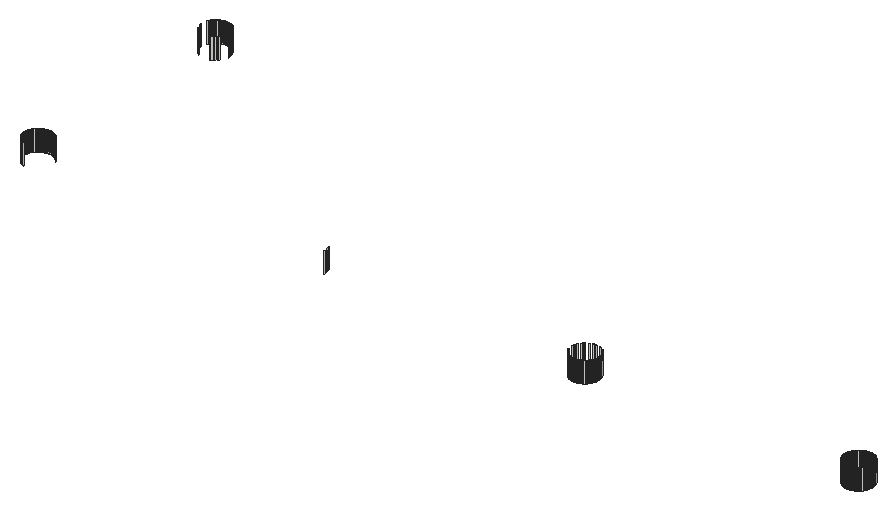
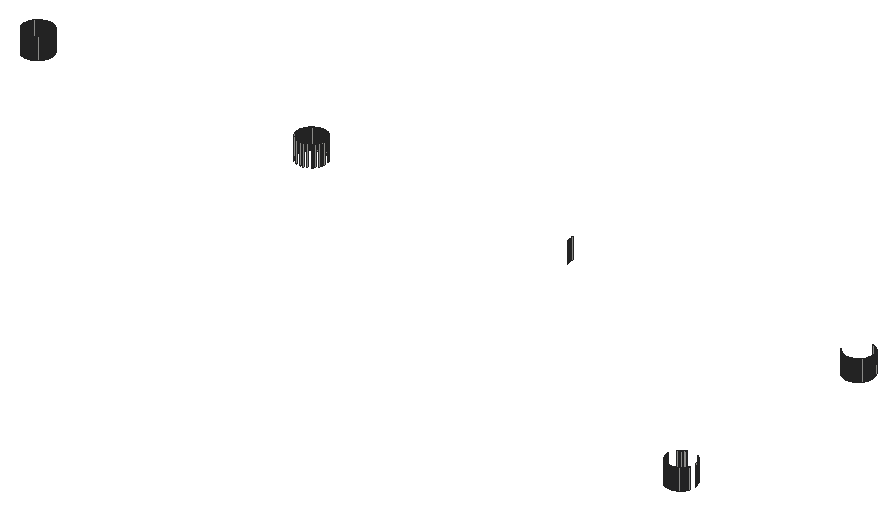
# SketchUp Ruby script. Lengths in millimetres.
U = 1.mm
M = Sketchup.active_model
def pt(a) = Geom::Point3d.new(a.map { |v| v * U })
def face(e, loops, mat)
  f = e.add_face(loops[0].map { |a| pt(a) })
  loops[1..].each { |l| e.add_face(l.map { |a| pt(a) }).erase! }
  f.material = f.back_material = mat if mat
  f
end
# faces: each face lists its corners as indices into pts; further lists are holes
def faces(e, pts, list, mat = nil) = list.each { |f| face(e, (f[0].is_a?(Array) ? f : [f]).map { |l| l.map { |i| pts[i] } }, mat) }
# xy, xz, yz: faces in a plane at the given z, y or x. An outline is a flat list of corners, or four numbers for a rectangle; further outlines are holes
def ring(l) = l.size == 4 ? [[l[0], l[1]], [l[2], l[1]], [l[2], l[3]], [l[0], l[3]]] : l.each_slice(2).to_a
def flat(e, list, mat, &to3) = list.each { |f| face(e, (f[0].is_a?(Array) ? f : [f]).map { |l| ring(l).map { |u, v| to3.(u, v) } }, mat) }
def xy(e, z, list, mat = nil) = flat(e, list, mat) { |x, y| [x, y, z] }
def xz(e, y, list, mat = nil) = flat(e, list, mat) { |x, z| [x, y, z] }
def yz(e, x, list, mat = nil) = flat(e, list, mat) { |y, z| [x, y, z] }
def lines(e, pts, list) = list.each { |a, b| e.add_line(pt(pts[a]), pt(pts[b])) }
# prism: a flat outline (further loops are holes) pulled along v
def prism(e, loops, v, mat = nil)
  f = face(e, loops, mat); d = Geom::Vector3d.new(v.map { |x| x * U })
  f.pushpull(f.normal.samedirection?(d) ? d.length : -d.length)
end
def box(e, o, s, mat = nil) = prism(e, [[o, [o[0] + s[0], o[1], o[2]], [o[0] + s[0], o[1] + s[1], o[2]], [o[0], o[1] + s[1], o[2]]]], [0, 0, s[2]], mat)
def at(x, y, z, deg = 0) = Geom::Transformation.translation(pt([x, y, z])) * Geom::Transformation.rotation(ORIGIN, Z_AXIS, deg.degrees)
def axes(o, x, y, z) = Geom::Transformation.new([*x, 0, *y, 0, *z, 0, *pt(o).to_a, 1])
def part(name) = M.definitions.add(name)
# library, detail: a bought-in or finely detailed component or shape, given as its bounding box
def library(name, o, s) = part(name).tap { |d| box(d.entities, o, s) }
def detail(e, o, s) = box(e.add_group.entities, o, s)
def put(e, d, t, mat = nil) = e.add_instance(d, t).tap { |i| i.material = mat if mat }
def group(e, t, mat = nil) = e.add_group.tap { |g| g.transformation = t; g.material = mat if mat }.entities
root = M.entities
p = [[2470.7,177.9,2718.2],[2470.7,177.9,2794],[2473.9,177.8,2794],[2473.9,177.8,2718.2],[2477.1,177.9,2794],[2477.1,177.9,2718.2],
  [3479,177.9,2718.2],[3479,177.9,2794],[3482.2,177.8,2794],[3482.2,177.8,2718.2],[3485.4,177.9,2794],[3485.4,177.9,2718.2],
  [2467.5,178.2,2718.2],[2467.5,178.2,2794],[2480.2,178.2,2794],[2480.2,178.2,2718.2],[3475.8,178.2,2718.2],[3475.8,178.2,2794],
  [3488.6,178.2,2794],[3488.6,178.2,2718.2],[2464.3,178.7,2718.2],[2464.3,178.7,2794],[2483.4,178.7,2794],[2483.4,178.7,2718.2],
  [3472.7,178.7,2718.2],[3472.7,178.7,2794],[3491.7,178.7,2794],[3491.7,178.7,2718.2],[2461.2,179.4,2718.2],[2461.2,179.4,2794],
  [2486.5,179.4,2794],[2486.5,179.4,2718.2],[3469.6,179.4,2718.2],[3469.6,179.4,2794],[3494.8,179.4,2794],[3494.8,179.4,2718.2],
  [444.6,179.4,2794],[444.6,179.4,2718.2],[441.5,180.3,2718.2],[441.5,180.3,2794],[2458.2,180.3,2718.2],[2458.2,180.3,2794],
  [2489.6,180.3,2794],[2489.6,180.3,2718.2],[3466.5,180.3,2718.2],[3466.5,180.3,2794],[3497.9,180.3,2794],[3497.9,180.3,2718.2],
  [438.5,181.4,2718.2],[438.5,181.4,2794],[2455.2,181.4,2718.2],[2455.2,181.4,2794],[2492.6,181.4,2794],[2492.6,181.4,2718.2],
  [3463.5,181.4,2718.2],[3463.5,181.4,2794],[3500.9,181.4,2794],[3500.9,181.4,2718.2],[435.6,182.6,2718.2],[435.6,182.6,2794],
  [2452.2,182.6,2718.2],[2452.2,182.6,2794],[2495.5,182.6,2794],[2495.5,182.6,2718.2],[3460.6,182.6,2718.2],[3460.6,182.6,2794],
  [3503.8,182.6,2794],[3503.8,182.6,2718.2],[432.7,184.1,2718.2],[432.7,184.1,2794],[2449.4,184.1,2718.2],[2449.4,184.1,2794],
  [2498.3,184.1,2794],[2498.3,184.1,2718.2],[3457.7,184.1,2718.2],[3457.7,184.1,2794],[3506.7,184.1,2794],[3506.7,184.1,2718.2],
  [430,185.7,2718.2],[430,185.7,2794],[2446.6,185.7,2718.2],[2446.6,185.7,2794],[2501.1,185.7,2794],[2501.1,185.7,2718.2],
  [3455,185.7,2718.2],[3455,185.7,2794],[3509.4,185.7,2794],[3509.4,185.7,2718.2],[427.3,187.5,2718.2],[427.3,187.5,2794],
  [2444,187.5,2718.2],[2444,187.5,2794],[2503.7,187.5,2794],[2503.7,187.5,2718.2],[3452.3,187.5,2718.2],[3452.3,187.5,2794],
  [3512.1,187.5,2794],[3512.1,187.5,2718.2],[424.8,189.5,2718.2],[424.8,189.5,2794],[2441.5,189.5,2718.2],[2441.5,189.5,2794],
  [2506.2,189.5,2794],[2506.2,189.5,2718.2],[3449.8,189.5,2718.2],[3449.8,189.5,2794],[3514.6,189.5,2794],[3514.6,189.5,2718.2],
  [422.4,191.6,2718.2],[422.4,191.6,2794],[2439.1,191.6,2718.2],[2439.1,191.6,2794],[2508.6,191.6,2794],[2508.6,191.6,2718.2],
  [3447.4,191.6,2718.2],[3447.4,191.6,2794],[3517,191.6,2794],[3517,191.6,2718.2],[420.2,193.8,2718.2],[420.2,193.8,2794],
  [2436.8,193.8,2718.2],[2436.8,193.8,2794],[2510.9,193.8,2794],[2510.9,193.8,2718.2],[3445.2,193.8,2718.2],[3445.2,193.8,2794],
  [3519.2,193.8,2794],[3519.2,193.8,2718.2],[418.1,196.2,2718.2],[418.1,196.2,2794],[2434.7,196.2,2718.2],[2434.7,196.2,2794],
  [2513,196.2,2794],[2513,196.2,2718.2],[3443.1,196.2,2718.2],[3443.1,196.2,2794],[3521.3,196.2,2794],[3521.3,196.2,2718.2],
  [416.1,198.7,2718.2],[416.1,198.7,2794],[2432.8,198.7,2718.2],[2432.8,198.7,2794],[2515,198.7,2794],[2515,198.7,2718.2],
  [3441.1,198.7,2718.2],[3441.1,198.7,2794],[3523.3,198.7,2794],[3523.3,198.7,2718.2],[414.3,201.4,2718.2],[414.3,201.4,2794],
  [2431,201.4,2718.2],[2431,201.4,2794],[2516.8,201.4,2794],[2516.8,201.4,2718.2],[3439.3,201.4,2718.2],[3439.3,201.4,2794],
  [3525.1,201.4,2794],[3525.1,201.4,2718.2],[412.7,204.1,2718.2],[412.7,204.1,2794],[2429.4,204.1,2718.2],[2429.4,204.1,2794],
  [2518.4,204.1,2794],[2518.4,204.1,2718.2],[3437.7,204.1,2718.2],[3437.7,204.1,2794],[3526.7,204.1,2794],[3526.7,204.1,2718.2],
  [411.2,207,2718.2],[411.2,207,2794],[2427.9,207,2718.2],[2427.9,207,2794],[2519.8,207,2794],[2519.8,207,2718.2],
  [3436.2,207,2718.2],[3436.2,207,2794],[3528.2,207,2794],[3528.2,207,2718.2],[410,209.9,2718.2],[410,209.9,2794],
  [2426.6,209.9,2718.2],[2426.6,209.9,2794],[2521.1,209.9,2794],[2521.1,209.9,2718.2],[3435,209.9,2718.2],[3435,209.9,2794],
  [3529.4,209.9,2794],[3529.4,209.9,2718.2],[408.9,212.9,2718.2],[408.9,212.9,2794],[2425.6,212.9,2718.2],[2425.6,212.9,2794],
  [2522.2,212.9,2794],[2522.2,212.9,2718.2],[3433.9,212.9,2718.2],[3433.9,212.9,2794],[3530.5,212.9,2794],[3530.5,212.9,2718.2],
  [408,216,2718.2],[408,216,2794],[2523.1,216,2794],[2523.1,216,2718.2],[3433,216,2718.2],[3433,216,2794],
  [3531.4,216,2794],[3531.4,216,2718.2],[407.3,219.1,2718.2],[407.3,219.1,2794],[2523.8,219.1,2794],[2523.8,219.1,2718.2],
  [3432.3,219.1,2718.2],[3432.3,219.1,2794],[3532.1,219.1,2794],[3532.1,219.1,2718.2],[406.8,222.2,2718.2],[406.8,222.2,2794],
  [2524.3,222.2,2794],[2524.3,222.2,2718.2],[3431.8,222.2,2718.2],[3431.8,222.2,2794],[3532.6,222.2,2794],[3532.6,222.2,2718.2],
  [406.5,225.4,2718.2],[406.5,225.4,2794],[1516.2,225.4,2794],[1516.2,225.4,2718.2],[1515.9,222.2,2718.2],[1515.9,222.2,2794],
  [2524.6,225.4,2794],[2524.6,225.4,2718.2],[3431.5,225.4,2718.2],[3431.5,225.4,2794],[3532.9,225.4,2794],[3532.9,225.4,2718.2],
  [406.4,228.6,2718.2],[406.4,228.6,2794],[2524.7,228.6,2794],[2524.7,228.6,2718.2],[3431.4,228.6,2718.2],[3431.4,228.6,2794],
  [3533,228.6,2794],[3533,228.6,2718.2],[406.5,231.8,2718.2],[406.5,231.8,2794],[2524.6,231.8,2794],[2524.6,231.8,2718.2],
  [3431.5,231.8,2718.2],[3431.5,231.8,2794],[3532.9,231.8,2794],[3532.9,231.8,2718.2],[406.8,235,2718.2],[406.8,235,2794],
  [2423.2,231.8,2794],[2423.2,231.8,2718.2],[2423.5,235,2718.2],[2423.5,235,2794],[2524.3,235,2794],[2524.3,235,2718.2],
  [3431.8,235,2718.2],[3431.8,235,2794],[3532.6,235,2794],[3532.6,235,2718.2],[407.3,238.1,2718.2],[407.3,238.1,2794],
  [2424,238.1,2718.2],[2424,238.1,2794],[2523.8,238.1,2794],[2523.8,238.1,2718.2],[3432.3,238.1,2718.2],[3432.3,238.1,2794],
  [3532.1,238.1,2794],[3532.1,238.1,2718.2],[408,241.2,2718.2],[408,241.2,2794],[1514.7,241.2,2794],[1514.7,241.2,2718.2],
  [1515.4,238.1,2718.2],[1515.4,238.1,2794],[2424.7,241.2,2718.2],[2424.7,241.2,2794],[2523.1,241.2,2794],[2523.1,241.2,2718.2],
  [3433,241.2,2718.2],[3433,241.2,2794],[3531.4,241.2,2794],[3531.4,241.2,2718.2],[408.9,244.3,2718.2],[408.9,244.3,2794],
  [1513.8,244.3,2794],[1513.8,244.3,2718.2],[2522.2,244.3,2794],[2522.2,244.3,2718.2],[3433.9,244.3,2718.2],[3433.9,244.3,2794],
  [3530.5,244.3,2794],[3530.5,244.3,2718.2],[410,247.3,2718.2],[410,247.3,2794],[1512.8,247.3,2794],[1512.8,247.3,2718.2],
  [2521.1,247.3,2794],[2521.1,247.3,2718.2],[3435,247.3,2718.2],[3435,247.3,2794],[3529.4,247.3,2794],[3529.4,247.3,2718.2],
  [411.2,250.2,2718.2],[411.2,250.2,2794],[1511.5,250.2,2794],[1511.5,250.2,2718.2],[2426.6,247.3,2794],[2426.6,247.3,2718.2],
  [2427.9,250.2,2718.2],[2427.9,250.2,2794],[2519.8,250.2,2794],[2519.8,250.2,2718.2],[3436.2,250.2,2718.2],[3436.2,250.2,2794],
  [3528.2,250.2,2794],[3528.2,250.2,2718.2],[412.7,253.1,2718.2],[412.7,253.1,2794],[2518.4,253.1,2794],[2518.4,253.1,2718.2],
  [3437.7,253.1,2718.2],[3437.7,253.1,2794],[3526.7,253.1,2794],[3526.7,253.1,2718.2],[414.3,255.8,2718.2],[414.3,255.8,2794],
  [500.1,255.8,2794],[500.1,255.8,2718.2],[501.7,253.1,2718.2],[501.7,253.1,2794],[3439.3,255.8,2718.2],[3439.3,255.8,2794],
  [3525.1,255.8,2794],[3525.1,255.8,2718.2],[416.1,258.5,2718.2],[416.1,258.5,2794],[498.3,258.5,2794],[498.3,258.5,2718.2],
  [3441.1,258.5,2718.2],[3441.1,258.5,2794],[3523.3,258.5,2794],[3523.3,258.5,2718.2],[418.1,261,2718.2],[418.1,261,2794],
  [496.3,261,2794],[496.3,261,2718.2],[2432.8,258.5,2794],[2432.8,258.5,2718.2],[2434.7,261,2718.2],[2434.7,261,2794],
  [3443.1,261,2718.2],[3443.1,261,2794],[3521.3,261,2794],[3521.3,261,2718.2],[420.2,263.4,2718.2],[420.2,263.4,2794],
  [494.2,263.4,2794],[494.2,263.4,2718.2],[2436.8,263.4,2718.2],[2436.8,263.4,2794],[3445.2,263.4,2718.2],[3445.2,263.4,2794],
  [3519.2,263.4,2794],[3519.2,263.4,2718.2],[422.4,265.6,2718.2],[422.4,265.6,2794],[492,265.6,2794],[492,265.6,2718.2],
  [2439.1,265.6,2718.2],[2439.1,265.6,2794],[3447.4,265.6,2718.2],[3447.4,265.6,2794],[3517,265.6,2794],[3517,265.6,2718.2],
  [424.8,267.7,2718.2],[424.8,267.7,2794],[489.6,267.7,2794],[489.6,267.7,2718.2],[2441.5,267.7,2718.2],[2441.5,267.7,2794],
  [2506.2,267.7,2794],[2506.2,267.7,2718.2],[2508.6,265.6,2718.2],[2508.6,265.6,2794],[3449.8,267.7,2718.2],[3449.8,267.7,2794],
  [3514.6,267.7,2794],[3514.6,267.7,2718.2],[427.3,269.7,2718.2],[427.3,269.7,2794],[487.1,269.7,2794],[487.1,269.7,2718.2],
  [3452.3,269.7,2718.2],[3452.3,269.7,2794],[3512.1,269.7,2794],[3512.1,269.7,2718.2],[430,271.5,2718.2],[430,271.5,2794],
  [484.4,271.5,2794],[484.4,271.5,2718.2],[3455,271.5,2718.2],[3455,271.5,2794],[3509.4,271.5,2794],[3509.4,271.5,2718.2],
  [432.7,273.1,2718.2],[432.7,273.1,2794],[481.7,273.1,2794],[481.7,273.1,2718.2],[3457.7,273.1,2718.2],[3457.7,273.1,2794],
  [3506.7,273.1,2794],[3506.7,273.1,2718.2],[435.6,274.6,2718.2],[435.6,274.6,2794],[478.8,274.6,2794],[478.8,274.6,2718.2],
  [3460.6,274.6,2718.2],[3460.6,274.6,2794],[3503.8,274.6,2794],[3503.8,274.6,2718.2],[438.5,275.8,2718.2],[438.5,275.8,2794],
  [475.9,275.8,2794],[475.9,275.8,2718.2],[2452.2,274.6,2794],[2452.2,274.6,2718.2],[2455.2,275.8,2718.2],[2455.2,275.8,2794],
  [3463.5,275.8,2718.2],[3463.5,275.8,2794],[3500.9,275.8,2794],[3500.9,275.8,2718.2],[441.5,276.9,2718.2],[441.5,276.9,2794],
  [472.9,276.9,2794],[472.9,276.9,2718.2],[2489.6,276.9,2794],[2489.6,276.9,2718.2],[2492.6,275.8,2718.2],[2492.6,275.8,2794],
  [3466.5,276.9,2718.2],[3466.5,276.9,2794],[3497.9,276.9,2794],[3497.9,276.9,2718.2],[444.6,277.8,2718.2],[444.6,277.8,2794],
  [469.8,277.8,2794],[469.8,277.8,2718.2],[3469.6,277.8,2718.2],[3469.6,277.8,2794],[3494.8,277.8,2794],[3494.8,277.8,2718.2],
  [447.7,278.5,2718.2],[447.7,278.5,2794],[466.7,278.5,2794],[466.7,278.5,2718.2],[2461.2,277.8,2794],[2461.2,277.8,2718.2],
  [2464.3,278.5,2718.2],[2464.3,278.5,2794],[3472.7,278.5,2718.2],[3472.7,278.5,2794],[3491.7,278.5,2794],[3491.7,278.5,2718.2],
  [450.8,279,2718.2],[450.8,279,2794],[463.6,279,2794],[463.6,279,2718.2],[2467.5,279,2718.2],[2467.5,279,2794],
  [3475.8,279,2718.2],[3475.8,279,2794],[3488.6,279,2794],[3488.6,279,2718.2],[454,279.3,2718.2],[454,279.3,2794],
  [460.4,279.3,2794],[460.4,279.3,2718.2],[3479,279.3,2718.2],[3479,279.3,2794],[3485.4,279.3,2794],[3485.4,279.3,2718.2],
  [457.2,279.4,2718.2],[457.2,279.4,2794],[2473.9,279.4,2794],[2473.9,279.4,2718.2],[2477.1,279.3,2718.2],[2477.1,279.3,2794],
  [3482.2,279.4,2718.2],[3482.2,279.4,2794],[475.9,999,2718.2],[475.9,999,2794],[478.8,1000.3,2794],[478.8,1000.3,2718.2],
  [481.7,1001.8,2794],[481.7,1001.8,2718.2],[430,1003.4,2718.2],[430,1003.4,2794],[432.7,1001.8,2794],[432.7,1001.8,2718.2],
  [427.3,1005.2,2718.2],[427.3,1005.2,2794],[484.4,1003.4,2718.2],[484.4,1003.4,2794],[487.1,1005.2,2794],[487.1,1005.2,2718.2],
  [489.6,1007.1,2794],[489.6,1007.1,2718.2],[422.4,1009.2,2718.2],[422.4,1009.2,2794],[424.8,1007.1,2794],[424.8,1007.1,2718.2],
  [420.2,1011.5,2718.2],[420.2,1011.5,2794],[494.2,1011.5,2718.2],[494.2,1011.5,2794],[496.3,1013.9,2794],[496.3,1013.9,2718.2],
  [416.1,1016.4,2718.2],[416.1,1016.4,2794],[418.1,1013.9,2794],[418.1,1013.9,2718.2],[498.3,1016.4,2794],[498.3,1016.4,2718.2],
  [414.3,1019,2718.2],[414.3,1019,2794],[407.3,1036.7,2718.2],[407.3,1036.7,2794],[408,1033.6,2794],[408,1033.6,2718.2],
  [406.8,1039.9,2718.2],[406.8,1039.9,2794],[507.9,1043.1,2718.2],[507.9,1043.1,2794],[508,1046.3,2794],[508,1046.3,2718.2],
  [507.9,1049.5,2794],[507.9,1049.5,2718.2],[507.6,1052.6,2794],[507.6,1052.6,2718.2],[507.1,1055.8,2794],[507.1,1055.8,2718.2],
  [506.4,1058.9,2794],[506.4,1058.9,2718.2],[505.5,1062,2794],[505.5,1062,2718.2],[504.4,1065,2794],[504.4,1065,2718.2],
  [411.2,1067.9,2718.2],[411.2,1067.9,2794],[410,1065,2794],[410,1065,2718.2],[412.7,1070.7,2718.2],[412.7,1070.7,2794],
  [414.3,1073.5,2718.2],[414.3,1073.5,2794],[501.7,1070.7,2718.2],[501.7,1070.7,2794],[500.1,1073.5,2794],[500.1,1073.5,2718.2],
  [416.1,1076.1,2718.2],[416.1,1076.1,2794],[498.3,1076.1,2794],[498.3,1076.1,2718.2],[418.1,1078.6,2718.2],[418.1,1078.6,2794],
  [496.3,1078.6,2794],[496.3,1078.6,2718.2],[420.2,1081,2718.2],[420.2,1081,2794],[494.2,1081,2794],[494.2,1081,2718.2],
  [422.4,1083.3,2718.2],[422.4,1083.3,2794],[492,1083.3,2794],[492,1083.3,2718.2],[424.8,1085.4,2718.2],[424.8,1085.4,2794],
  [489.6,1085.4,2794],[489.6,1085.4,2718.2],[427.3,1087.4,2718.2],[427.3,1087.4,2794],[487.1,1087.4,2794],[487.1,1087.4,2718.2],
  [430,1089.2,2718.2],[430,1089.2,2794],[484.4,1089.2,2794],[484.4,1089.2,2718.2],[432.7,1090.8,2718.2],[432.7,1090.8,2794],
  [481.7,1090.8,2794],[481.7,1090.8,2718.2],[435.6,1092.2,2718.2],[435.6,1092.2,2794],[478.8,1092.2,2794],[478.8,1092.2,2718.2],
  [438.5,1093.5,2718.2],[438.5,1093.5,2794],[475.9,1093.5,2794],[475.9,1093.5,2718.2],[441.5,1094.6,2718.2],[441.5,1094.6,2794],
  [472.9,1094.6,2794],[472.9,1094.6,2718.2],[444.6,1095.5,2718.2],[444.6,1095.5,2794],[469.8,1095.5,2794],[469.8,1095.5,2718.2],
  [447.7,1096.2,2718.2],[447.7,1096.2,2794],[466.7,1096.2,2794],[466.7,1096.2,2718.2],[450.8,1096.7,2718.2],[450.8,1096.7,2794],
  [463.6,1096.7,2794],[463.6,1096.7,2718.2],[454,1097,2718.2],[454,1097,2794],[460.4,1097,2794],[460.4,1097,2718.2],
  [457.2,1097.1,2718.2],[457.2,1097.1,2794]]
faces(root,p,[[0,1,2,3],[3,2,4,5],[6,7,8,9],[9,8,10,11],[12,13,1,0],[5,4,14,15],[16,17,7,6],[11,10,18,19],
  [20,21,13,12],[15,14,22,23],[24,25,17,16],[19,18,26,27],[28,29,21,20],[23,22,30,31],[32,33,25,24],[27,26,34,35],
  [36,37,38,39],[40,41,29,28],[31,30,42,43],[44,45,33,32],[35,34,46,47],[39,38,48,49],[50,51,41,40],[43,42,52,53],
  [54,55,45,44],[47,46,56,57],[49,48,58,59],[60,61,51,50],[53,52,62,63],[64,65,55,54],[57,56,66,67],[59,58,68,69],
  [70,71,61,60],[63,62,72,73],[74,75,65,64],[67,66,76,77],[69,68,78,79],[80,81,71,70],[73,72,82,83],[84,85,75,74],
  [77,76,86,87],[79,78,88,89],[90,91,81,80],[83,82,92,93],[94,95,85,84],[87,86,96,97],[89,88,98,99],[100,101,91,90],
  [93,92,102,103],[104,105,95,94],[97,96,106,107],[99,98,108,109],[110,111,101,100],[103,102,112,113],[114,115,105,104],[107,106,116,117],
  [109,108,118,119],[120,121,111,110],[113,112,122,123],[124,125,115,114],[117,116,126,127],[119,118,128,129],[130,131,121,120],[123,122,132,133],
  [134,135,125,124],[127,126,136,137],[129,128,138,139],[140,141,131,130],[133,132,142,143],[144,145,135,134],[137,136,146,147],[139,138,148,149],
  [150,151,141,140],[143,142,152,153],[154,155,145,144],[147,146,156,157],[149,148,158,159],[160,161,151,150],[153,152,162,163],[164,165,155,154],
  [157,156,166,167],[159,158,168,169],[170,171,161,160],[163,162,172,173],[174,175,165,164],[167,166,176,177],[169,168,178,179],[180,181,171,170],
  [173,172,182,183],[184,185,175,174],[177,176,186,187],[179,178,188,189],[190,191,181,180],[183,182,192,193],[194,195,185,184],[187,186,196,197],
  [189,188,198,199],[193,192,200,201],[202,203,195,194],[197,196,204,205],[199,198,206,207],[201,200,208,209],[210,211,203,202],[205,204,212,213],
  [207,206,214,215],[209,208,216,217],[218,219,211,210],[213,212,220,221],[215,214,222,223],[224,225,226,227],[217,216,228,229],[230,231,219,218],
  [221,220,232,233],[223,222,234,235],[236,237,229,228],[238,239,231,230],[233,232,240,241],[235,234,242,243],[244,245,237,236],[246,247,239,238],
  [241,240,248,249],[243,242,250,251],[252,253,254,255],[256,257,245,244],[258,259,247,246],[249,248,260,261],[251,250,262,263],[255,254,264,265],
  [257,256,266,267],[268,269,259,258],[261,260,270,271],[263,262,272,273],[274,275,276,277],[265,264,278,279],[267,266,280,281],[282,283,269,268],
  [271,270,284,285],[273,272,286,287],[288,289,275,274],[281,280,290,291],[292,293,283,282],[285,284,294,295],[287,286,296,297],[298,299,289,288],
  [291,290,300,301],[302,303,293,292],[295,294,304,305],[297,296,306,307],[308,309,299,298],[310,311,312,313],[301,300,314,315],[316,317,303,302],
  [305,304,318,319],[307,306,320,321],[315,314,322,323],[324,325,317,316],[319,318,326,327],[321,320,328,329],[330,331,332,333],[334,335,325,324],
  [327,326,336,337],[329,328,338,339],[340,341,331,330],[342,343,335,334],[337,336,344,345],[339,338,346,347],[348,349,341,340],[350,351,352,353],
  [354,355,343,342],[345,344,356,357],[347,346,358,359],[360,361,349,348],[353,352,362,363],[364,365,355,354],[357,356,366,367],[359,358,368,369],
  [370,371,361,360],[363,362,372,373],[374,375,365,364],[367,366,376,377],[369,368,378,379],[380,381,371,370],[373,372,382,383],[384,385,386,387],
  [388,389,375,374],[377,376,390,391],[379,378,392,393],[394,395,381,380],[396,397,389,388],[391,390,398,399],[393,392,400,401],[402,403,395,394],
  [404,405,397,396],[399,398,406,407],[401,400,408,409],[410,411,403,402],[412,413,405,404],[407,406,414,415],[409,408,416,417],[418,419,411,410],
  [420,421,413,412],[415,414,422,423],[417,416,424,425],[426,427,419,418],[428,429,430,431],[432,433,421,420],[423,422,434,435],[425,424,436,437],
  [438,439,427,426],[440,441,442,443],[444,445,433,432],[435,434,446,447],[437,436,448,449],[450,451,439,438],[452,453,445,444],[447,446,454,455],
  [449,448,456,457],[458,459,451,450],[460,461,462,463],[464,465,453,452],[455,454,466,467],[457,456,468,469],[470,471,459,458],[463,462,472,473],
  [474,475,465,464],[467,466,476,477],[469,468,478,479],[480,481,471,470],[482,483,475,474],[477,476,484,485],[479,478,486,487],[487,486,481,480],
  [488,489,490,491],[492,493,483,482],[485,484,493,492],[494,495,496,497],[497,496,498,499],[500,501,502,503],[504,505,501,500],[506,507,508,509],
  [509,508,510,511],[512,513,514,515],[516,517,513,512],[518,519,520,521],[522,523,524,525],[521,520,526,527],[528,529,523,522],[530,531,532,533],
  [534,535,531,530],[536,537,538,539],[539,538,540,541],[541,540,542,543],[543,542,544,545],[545,544,546,547],[547,546,548,549],[549,548,550,551],
  [552,553,554,555],[556,557,553,552],[558,559,557,556],[560,561,562,563],[564,565,559,558],[563,562,566,567],[568,569,565,564],[567,566,570,571],
  [572,573,569,568],[571,570,574,575],[576,577,573,572],[575,574,578,579],[580,581,577,576],[579,578,582,583],[584,585,581,580],[583,582,586,587],
  [588,589,585,584],[587,586,590,591],[592,593,589,588],[591,590,594,595],[596,597,593,592],[595,594,598,599],[600,601,597,596],[599,598,602,603],
  [604,605,601,600],[603,602,606,607],[608,609,605,604],[607,606,610,611],[612,613,609,608],[611,610,614,615],[616,617,613,612],[615,614,618,619],
  [620,621,617,616],[619,618,622,623],[624,625,621,620],[623,622,625,624]])
